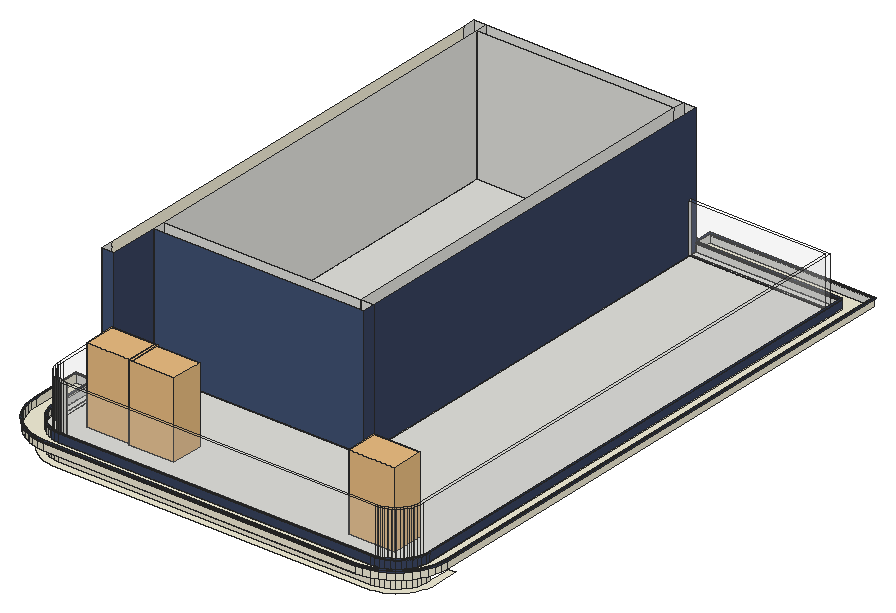
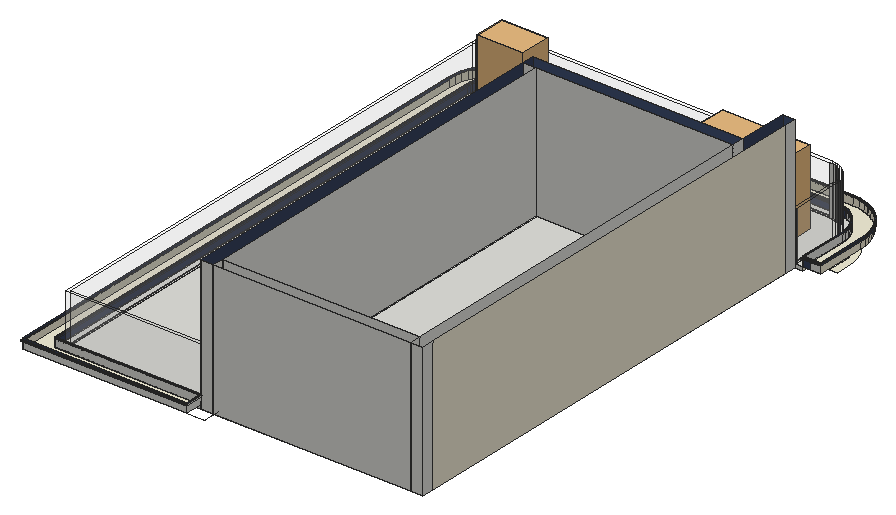
# SketchUp Ruby script. Lengths in inches.
U = 1.inch
M = Sketchup.active_model
def pt(a) = Geom::Point3d.new(a.map { |v| v * U })
def face(e, loops, mat)
  f = e.add_face(loops[0].map { |a| pt(a) })
  loops[1..].each { |l| e.add_face(l.map { |a| pt(a) }).erase! }
  f.material = f.back_material = mat if mat
  f
end
# faces: each face lists its corners as indices into pts; further lists are holes
def faces(e, pts, list, mat = nil) = list.each { |f| face(e, (f[0].is_a?(Array) ? f : [f]).map { |l| l.map { |i| pts[i] } }, mat) }
# xy, xz, yz: faces in a plane at the given z, y or x. An outline is a flat list of corners, or four numbers for a rectangle; further outlines are holes
def ring(l) = l.size == 4 ? [[l[0], l[1]], [l[2], l[1]], [l[2], l[3]], [l[0], l[3]]] : l.each_slice(2).to_a
def flat(e, list, mat, &to3) = list.each { |f| face(e, (f[0].is_a?(Array) ? f : [f]).map { |l| ring(l).map { |u, v| to3.(u, v) } }, mat) }
def xy(e, z, list, mat = nil) = flat(e, list, mat) { |x, y| [x, y, z] }
def xz(e, y, list, mat = nil) = flat(e, list, mat) { |x, z| [x, y, z] }
def yz(e, x, list, mat = nil) = flat(e, list, mat) { |y, z| [x, y, z] }
def lines(e, pts, list) = list.each { |a, b| e.add_line(pt(pts[a]), pt(pts[b])) }
# prism: a flat outline (further loops are holes) pulled along v
def prism(e, loops, v, mat = nil)
  f = face(e, loops, mat); d = Geom::Vector3d.new(v.map { |x| x * U })
  f.pushpull(f.normal.samedirection?(d) ? d.length : -d.length)
end
def box(e, o, s, mat = nil) = prism(e, [[o, [o[0] + s[0], o[1], o[2]], [o[0] + s[0], o[1] + s[1], o[2]], [o[0], o[1] + s[1], o[2]]]], [0, 0, s[2]], mat)
def at(x, y, z, deg = 0) = Geom::Transformation.translation(pt([x, y, z])) * Geom::Transformation.rotation(ORIGIN, Z_AXIS, deg.degrees)
def axes(o, x, y, z) = Geom::Transformation.new([*x, 0, *y, 0, *z, 0, *pt(o).to_a, 1])
def part(name) = M.definitions.add(name)
# library, detail: a bought-in or finely detailed component or shape, given as its bounding box
def library(name, o, s) = part(name).tap { |d| box(d.entities, o, s) }
def detail(e, o, s) = box(e.add_group.entities, o, s)
def put(e, d, t, mat = nil) = e.add_instance(d, t).tap { |i| i.material = mat if mat }
def group(e, t, mat = nil) = e.add_group.tap { |g| g.transformation = t; g.material = mat if mat }.entities
root = M.entities
M.materials.add("0359 AP 9643 Sailor’s Stripes-N").color = [65, 82, 115]
M.materials.add("0360 AP 9644 Monsoon Midnight-N").color = [56, 67, 95]
M.materials.add("0905 AP 7844 MILD YELLOW").color = [242, 237, 215]
M.materials.add("Glass Clear 001").color = [246, 246, 246]
M.materials["Glass Clear 001"].alpha = 0.1
c1 = library("Ficus triangularis Variegata 002",[-17,-11.8,0.01],[33.04,22.7,54.61])
xy(root,253.9375,[[134.66,24.81,360,24.81,363.8,25.06,367.54,25.8,371.15,27.03,374.56,28.71,377.73,30.83,380.6,33.34,383.11,36.2,385.23,39.37,386.91,42.79,388.14,46.4,388.88,50.14,389.13,53.9375,389.13,71.07,384,71.07,384,53.9375,383.79,50.8,383.18,47.73,382.17,44.75,380.78,41.9375,379.04,39.33,376.97,36.97,374.61,34.9,372,33.15,369.18,31.76,366.21,30.76,363.13,30.14,360,29.9375,134.95,29.9375,131.9375,30.29,128.99,31.02,126.8125,31.86,126.15,32.11,123.48,33.56,121.01,35.33,118.78,37.4,116.84,39.73,115.2,42.29,113.9,45.03,112.95,47.92,112.38,50.91,112.1875,53.9375,112.1875,65.19,107.06,65.19,107.06,53.78,107.28,50.26,107.98,46.63,109.125,43.13,110.7,39.8,112.69,36.69,115.06,33.86,117.76,31.35,120.76,29.2,124,27.45,124.96,27.08,127.44,26.12,131.02,25.23]],"0905 AP 7844 MILD YELLOW")
xy(root,264,[[134.95,29.9375,131.9375,30.29,128.99,31.02,126.8125,31.86,126.15,32.11,123.48,33.56,121.01,35.33,118.78,37.4,116.84,39.73,115.2,42.29,113.9,45.03,112.95,47.92,112.38,50.91,112.1875,53.9375,112.1875,89.9375,126.8125,89.9375,126.8125,125.9375,278.3125,125.9375,278.3125,425.9375,384,425.9375,384,53.9375,383.79,50.8,383.18,47.73,382.17,44.75,380.78,41.9375,379.04,39.33,376.97,36.97,374.61,34.9,372,33.15,369.18,31.76,366.21,30.76,363.13,30.14,360,29.9375],[117.8125,89.9375,126.8125,425.9375],[126.8125,125.9375,278.3125,134.9375],[126.8125,134.9375,269.3125,417.55],[269.3125,134.9375,278.3125,425.9375],
  [126.8125,417.55,269.3125,425.9375]])
xy(root,266.6875,[[134.95,29.9375,360,29.9375,363.13,30.14,366.21,30.76,369.18,31.76,372,33.15,374.61,34.9,376.97,36.97,379.04,39.33,380.78,41.9375,382.17,44.75,383.18,47.73,383.79,50.8,384,53.9375,384,425.9375,278.3125,425.9375,278.3125,421.33,379.39,421.33,379.39,53.9375,379.23,51.41,378.73,48.92,377.92,46.52,376.79,44.24,375.39,42.13,373.71,40.23,371.81,38.55,369.7,37.14,367.42,36.02,365.02,35.21,362.53,34.71,360,34.55,135.22,34.55,132.76,34.83,130.375,35.42,128.47,36.16,128.09,36.31,125.93,37.47,123.93,38.9,122.13,40.57,120.5625,42.46,119.24,44.53,118.1875,46.74,117.42,49.08,116.96,51.49,116.8,54.08,116.8,89.9375,112.1875,89.9375,112.1875,53.9375,112.38,50.91,112.95,47.92,113.9,45.03,115.2,42.29,116.84,39.73,118.78,37.4,121.01,35.33,123.48,33.56,126.15,32.11,126.8125,31.86,128.99,31.02,131.9375,30.29],[135.22,34.55,132.76,34.83,130.375,35.42,128.47,36.16,128.09,36.31,125.93,37.47,123.93,38.9,122.13,40.57,120.5625,42.46,119.24,44.53,118.1875,46.74,117.42,49.08,116.96,51.49,116.8,54.08,116.8,89.9375,118.94,89.9375,118.94,54.15,119.09,51.76,119.5,49.62,120.18,47.54,121.12,45.57,122.29,43.73,123.69,42.05,125.29,40.57,127.07,39.3,128.99,38.26,129.25,38.16,131.02,37.47,133.14,36.95,135.35,36.69,360,36.69,362.25,36.84,364.46,37.28,366.6,38,368.625,39,370.5,40.25,372.2,41.74,373.68,43.4375,374.9375,45.3125,375.93,47.34,376.66,49.47,377.1,51.6875,377.25,53.9375,377.25,419.18,278.3125,419.18,278.3125,421.33,379.39,421.33,379.39,53.9375,379.23,51.41,378.73,48.92,377.92,46.52,376.79,44.24,375.39,42.13,373.71,40.23,371.81,38.55,369.7,37.14,367.42,36.02,365.02,35.21,362.53,34.71,360,34.55],[135.35,36.69,360,36.69,362.25,36.84,364.46,37.28,366.6,38,368.625,39,370.5,40.25,372.2,41.74,373.68,43.4375,374.9375,45.3125,375.93,47.34,376.66,49.47,377.1,51.6875,377.25,53.9375,377.25,419.18,278.3125,419.18,278.3125,125.9375,126.8125,125.9375,126.8125,89.9375,118.94,89.9375,118.94,54.15,119.09,51.76,119.5,49.62,120.18,47.54,121.12,45.57,122.29,43.73,123.69,42.05,125.29,40.57,127.07,39.3,128.99,38.26,129.25,38.16,131.02,37.47,133.14,36.95]])
xy(root,266.6875,[[134.21,17.08,129.64,17.61,125.11,18.73,122.17,19.87,120.76,20.42,116.65,22.63,112.86,25.35,109.4375,28.53,106.45,32.11,103.93,36.04,101.93,40.26,100.48,44.7,99.6,49.28,99.33,53.53,99.33,89.9375,112.1875,89.9375,112.1875,53.9375,112.38,50.91,112.95,47.92,113.9,45.03,115.2,42.29,116.84,39.73,118.78,37.4,121.01,35.33,123.48,33.56,126.15,32.11,126.8125,31.86,128.99,31.02,131.9375,30.29,134.95,29.9375,360,29.9375,363.13,30.14,366.21,30.76,369.18,31.76,372,33.15,374.61,34.9,376.97,36.97,379.04,39.33,380.78,41.9375,382.17,44.75,383.18,47.73,383.79,50.8,384,53.9375,384,425.9375,278.3125,425.9375,278.3125,438.8,396.86,438.8,396.86,53.9375,396.54,49.125,395.6,44.4,394.05,39.83,391.92,35.51,389.24,31.5,386.0625,27.875,382.4375,24.7,378.43,22.02,374.11,19.88,369.54,18.34,364.8125,17.39,360,17.08]],"0905 AP 7844 MILD YELLOW")
xy(root,272.125,[[[134.16,16.27,129.49,16.81,124.86,17.96,121.88,19.11,120.41,19.68,116.22,21.94,112.34,24.72,108.85,27.97,105.79,31.63,103.22,35.65,101.17,39.96,99.69,44.49,98.79,49.18,98.52,53.5,98.52,90.75,113,90.75,113,53.96,113.1875,51.01,113.74,48.125,114.65,45.34,115.91,42.68,117.49,40.21,119.375,37.96,121.53,35.96,123.91,34.25,126.49,32.85,127.11,32.62,129.23,31.8,132.08,31.09,135,30.75,360,30.75,363.03,30.95,366,31.54,368.875,32.52,371.59,33.86,374.12,35.54,376.4,37.54,378.4,39.82,380.08,42.34,381.42,45.0625,382.4,47.9375,382.99,50.91,383.1875,53.9375,383.1875,425.125,277.5,425.125,277.5,439.61,397.67,439.61,397.67,53.9375,397.35,49.02,396.39,44.1875,394.8,39.52,392.625,35.1,389.89,31,386.64,27.3,382.93,24.05,378.84,21.3125,374.42,19.13,369.75,17.55,364.92,16.59,360,16.27],[134.21,17.08,360,17.08,364.8125,17.39,369.54,18.34,374.11,19.88,378.43,22.02,382.4375,24.7,386.0625,27.875,389.24,31.5,391.92,35.51,394.05,39.83,395.6,44.4,396.54,49.125,396.86,53.9375,396.86,438.8,278.3125,438.8,278.3125,425.9375,384,425.9375,384,53.9375,383.79,50.8,383.18,47.73,382.17,44.75,380.78,41.9375,379.04,39.33,376.97,36.97,374.61,34.9,372,33.15,369.18,31.76,366.21,30.76,363.13,30.14,360,29.9375,134.95,29.9375,131.9375,30.29,128.99,31.02,126.8125,31.86,126.15,32.11,123.48,33.56,121.01,35.33,118.78,37.4,116.84,39.73,115.2,42.29,113.9,45.03,112.95,47.92,112.38,50.91,112.1875,53.9375,112.1875,89.9375,99.33,89.9375,99.33,53.53,99.6,49.28,100.48,44.7,101.93,40.26,103.93,36.04,106.45,32.11,109.4375,28.53,112.86,25.35,116.65,22.63,120.76,20.42,122.17,19.87,125.11,18.73,129.64,17.61]]],"0360 AP 9644 Monsoon Midnight-N")
xy(root,272.8125,[[[134.16,16.27,360,16.27,364.92,16.59,369.75,17.55,374.42,19.13,378.84,21.3125,382.93,24.05,386.64,27.3,389.89,31,392.625,35.1,394.8,39.52,396.39,44.1875,397.35,49.02,397.67,53.9375,397.67,439.61,277.5,439.61,277.5,425.125,383.1875,425.125,383.1875,53.9375,382.99,50.91,382.4,47.9375,381.42,45.0625,380.08,42.34,378.4,39.82,376.4,37.54,374.12,35.54,371.59,33.86,368.875,32.52,366,31.54,363.03,30.95,360,30.75,135,30.75,132.08,31.09,129.23,31.8,127.11,32.62,126.49,32.85,123.91,34.25,121.53,35.96,119.375,37.96,117.49,40.21,115.91,42.68,114.65,45.34,113.74,48.125,113.1875,51.01,113,53.96,113,90.75,98.52,90.75,98.52,53.5,98.79,49.18,99.69,44.49,101.17,39.96,103.22,35.65,105.79,31.63,108.85,27.97,112.34,24.72,116.22,21.94,120.41,19.68,121.88,19.11,124.86,17.96,129.49,16.81],[134.21,17.08,129.64,17.61,125.11,18.73,122.17,19.87,120.76,20.42,116.65,22.63,112.86,25.35,109.4375,28.53,106.45,32.11,103.93,36.04,101.93,40.26,100.48,44.7,99.6,49.28,99.33,53.53,99.33,89.9375,112.1875,89.9375,112.1875,53.9375,112.38,50.91,112.95,47.92,113.9,45.03,115.2,42.29,116.84,39.73,118.78,37.4,121.01,35.33,123.48,33.56,126.15,32.11,126.8125,31.86,128.99,31.02,131.9375,30.29,134.95,29.9375,360,29.9375,363.13,30.14,366.21,30.76,369.18,31.76,372,33.15,374.61,34.9,376.97,36.97,379.04,39.33,380.78,41.9375,382.17,44.75,383.18,47.73,383.79,50.8,384,53.9375,384,425.9375,278.3125,425.9375,278.3125,438.8,396.86,438.8,396.86,53.9375,396.54,49.125,395.6,44.4,394.05,39.83,391.92,35.51,389.24,31.5,386.0625,27.875,382.4375,24.7,378.43,22.02,374.11,19.88,369.54,18.34,364.8125,17.39,360,17.08]]],"0360 AP 9644 Monsoon Midnight-N")
xz(root,16.27,[[134.16,272.125,360,272.8125]],"0360 AP 9644 Monsoon Midnight-N")
xz(root,17.08,[[134.21,272.125,360,272.8125],[134.21,272.8125,360,273.625]],"0360 AP 9644 Monsoon Midnight-N")
xz(root,17.08,[[134.21,266.6875,360,272.125]],"0905 AP 7844 MILD YELLOW")
xz(root,29.9375,[[134.95,266.6875,360,272.125],[134.95,272.125,360,272.8125],[134.95,272.8125,360,273.625]],"0360 AP 9644 Monsoon Midnight-N")
xz(root,29.9375,[[134.95,253.9375,360,264],[134.95,264,360,266.6875]],"0905 AP 7844 MILD YELLOW")
xz(root,30.75,[[135,272.125,360,272.8125]],"0360 AP 9644 Monsoon Midnight-N")
xz(root,34.55,[[135.22,266.6875,360,302.6875]],"Glass Clear 001")
xz(root,36.69,[[135.35,266.6875,360,302.6875]],"Glass Clear 001")
xz(root,89.9375,[[112.1875,264,117.8125,266.6875],[117.8125,264,126.8125,266.6875],[99.33,266.6875,106.59,272.125],[116.8,266.6875,117.8125,302.6875],[117.8125,266.6875,118.94,302.6875],
  [106.59,272.125,112.1875,272.8125]])
xz(root,89.9375,[[118.94,266.6875,126.8125,266.6875,126.8125,360,117.8125,360,117.8125,303.4375,118.94,303.4375]],"0359 AP 9643 Sailor’s Stripes-N")
xz(root,89.9375,[[106.59,266.6875,112.1875,272.125],[99.33,272.125,106.59,272.8125],[99.33,272.8125,106.59,273.625],[106.59,272.8125,112.1875,273.625]],"0360 AP 9644 Monsoon Midnight-N")
xz(root,90.75,[[98.52,272.125,106.59,272.8125],[106.59,272.125,113,272.8125]])
xz(root,125.9375,[[126.8125,264,278.3125,266.6875]])
xz(root,125.9375,[[126.8125,266.6875,278.3125,360]],"0359 AP 9643 Sailor’s Stripes-N")
xz(root,134.9375,[[126.8125,264,269.3125,360],[269.3125,264,278.3125,360]])
xz(root,417.55,[[126.8125,264,269.3125,360]])
xz(root,419.18,[[278.3125,266.6875,377.25,302.6875]],"Glass Clear 001")
xz(root,421.33,[[278.3125,266.6875,379.39,302.6875]],"Glass Clear 001")
xz(root,425.125,[[277.5,272.125,383.1875,272.8125]])
xz(root,425.9375,[[117.8125,264,126.8125,360],[126.8125,264,269.3125,360],[269.3125,264,278.3125,360],[278.3125,264,384,266.6875],[278.3125,266.6875,384,272.125]])
xz(root,425.9375,[[278.3125,272.125,384,272.8125],[278.3125,272.8125,384,273.625]],"0360 AP 9644 Monsoon Midnight-N")
xz(root,438.8,[[278.3125,266.6875,396.86,272.125]])
xz(root,438.8,[[278.3125,272.125,396.86,272.8125],[278.3125,272.8125,396.86,273.625]],"0360 AP 9644 Monsoon Midnight-N")
xz(root,439.61,[[277.5,272.125,397.67,272.8125]])
yz(root,98.52,[[53.5,272.125,90.75,272.8125]],"0360 AP 9644 Monsoon Midnight-N")
yz(root,99.33,[[53.53,272.125,89.9375,272.8125],[53.53,272.8125,89.9375,273.625]],"0360 AP 9644 Monsoon Midnight-N")
yz(root,99.33,[[53.53,266.6875,89.9375,272.125]],"0905 AP 7844 MILD YELLOW")
yz(root,112.1875,[[53.9375,266.6875,89.9375,272.125]])
yz(root,112.1875,[[53.9375,272.125,89.9375,272.8125],[53.9375,272.8125,89.9375,273.625]],"0360 AP 9644 Monsoon Midnight-N")
yz(root,112.1875,[[53.9375,264,89.9375,266.6875]],"0905 AP 7844 MILD YELLOW")
yz(root,113,[[53.96,272.125,90.75,272.8125]])
yz(root,116.8,[[54.08,266.6875,89.9375,302.6875]],"Glass Clear 001")
yz(root,117.8125,[[89.9375,264,98.79,360],[416.9375,264,425.9375,360]])
yz(root,117.8125,[[98.79,264,416.9375,360]],"0905 AP 7844 MILD YELLOW")
yz(root,118.94,[[54.15,266.6875,89.9375,302.6875]],"Glass Clear 001")
yz(root,126.8125,[[89.9375,264,125.9375,266.6875],[125.9375,264,134.9375,360],[134.9375,264,417.55,360],[417.55,264,425.9375,360]])
yz(root,126.8125,[[89.9375,266.6875,125.9375,360]],"0360 AP 9644 Monsoon Midnight-N")
yz(root,269.3125,[[134.9375,264,417.55,360],[417.55,264,425.9375,360]])
yz(root,277.5,[[425.125,272.125,439.61,272.8125]])
yz(root,278.3125,[[125.9375,264,134.9375,266.6875],[134.9375,264,425.9375,266.6875],[419.18,266.6875,421.33,302.6875],[425.9375,266.6875,438.8,272.125]])
yz(root,278.3125,[[125.9375,266.6875,134.9375,360],[134.9375,266.6875,419.18,266.6875,419.18,303.4375,421.33,303.4375,421.33,266.6875,425.9375,266.6875,425.9375,360,134.9375,360],[425.9375,272.125,438.8,272.8125],[425.9375,272.8125,438.8,273.625]],"0360 AP 9644 Monsoon Midnight-N")
yz(root,377.25,[[53.9375,266.6875,419.18,302.6875]],"Glass Clear 001")
yz(root,379.39,[[53.9375,266.6875,421.33,302.6875]],"Glass Clear 001")
yz(root,383.1875,[[53.9375,272.125,425.125,272.8125]],"0360 AP 9644 Monsoon Midnight-N")
yz(root,384,[[53.9375,266.6875,425.9375,272.125],[53.9375,272.125,425.9375,272.8125],[53.9375,272.8125,425.9375,273.625]],"0360 AP 9644 Monsoon Midnight-N")
yz(root,384,[[53.9375,264,425.9375,266.6875]],"0905 AP 7844 MILD YELLOW")
yz(root,396.86,[[53.9375,272.125,438.8,272.8125],[53.9375,272.8125,438.8,273.625]],"0360 AP 9644 Monsoon Midnight-N")
yz(root,396.86,[[53.9375,266.6875,438.8,272.125]],"0905 AP 7844 MILD YELLOW")
yz(root,397.67,[[53.9375,272.125,439.61,272.8125]],"0360 AP 9644 Monsoon Midnight-N")
p = [[134.95,29.9375,264],[131.9375,30.29,264],[131.9375,30.29,253.9375],[134.95,29.9375,253.9375],[363.13,30.14,264],[360,29.9375,264],
  [360,29.9375,253.9375],[363.13,30.14,253.9375],[366.21,30.76,264],[366.21,30.76,253.9375],[128.99,31.02,264],[128.99,31.02,253.9375],
  [369.18,31.76,264],[369.18,31.76,253.9375],[126.8125,31.86,264],[126.8125,31.86,253.9375],[372,33.15,264],[372,33.15,253.9375],
  [126.15,32.11,264],[126.15,32.11,253.9375],[123.48,33.56,264],[123.48,33.56,253.9375],[374.61,34.9,264],[374.61,34.9,253.9375],
  [121.01,35.33,264],[121.01,35.33,253.9375],[376.97,36.97,264],[376.97,36.97,253.9375],[118.78,37.4,264],[118.78,37.4,253.9375],
  [379.04,39.33,264],[379.04,39.33,253.9375],[116.84,39.73,264],[116.84,39.73,253.9375],[380.78,41.9375,264],[380.78,41.9375,253.9375],
  [115.2,42.29,264],[115.2,42.29,253.9375],[382.17,44.75,264],[382.17,44.75,253.9375],[113.9,45.03,264],[113.9,45.03,253.9375],
  [383.18,47.73,264],[383.18,47.73,253.9375],[112.95,47.92,264],[112.95,47.92,253.9375],[383.79,50.8,264],[383.79,50.8,253.9375],
  [112.38,50.91,264],[112.38,50.91,253.9375],[384,53.9375,264],[384,53.9375,253.9375],[112.1875,53.9375,264],[112.1875,53.9375,253.9375],
  [134.95,29.9375,266.6875],[131.9375,30.29,266.6875],[363.13,30.14,266.6875],[360,29.9375,266.6875],[366.21,30.76,266.6875],[128.99,31.02,266.6875],
  [369.18,31.76,266.6875],[126.8125,31.86,266.6875],[372,33.15,266.6875],[126.15,32.11,266.6875],[123.48,33.56,266.6875],[374.61,34.9,266.6875],
  [121.01,35.33,266.6875],[376.97,36.97,266.6875],[118.78,37.4,266.6875],[379.04,39.33,266.6875],[116.84,39.73,266.6875],[380.78,41.9375,266.6875],
  [115.2,42.29,266.6875],[382.17,44.75,266.6875],[113.9,45.03,266.6875],[383.18,47.73,266.6875],[112.95,47.92,266.6875],[383.79,50.8,266.6875],
  [112.38,50.91,266.6875],[384,53.9375,266.6875],[112.1875,53.9375,266.6875],[129.64,17.61,266.6875],[134.21,17.08,266.6875],[134.21,17.08,272.125],
  [129.64,17.61,272.125],[360,17.08,266.6875],[364.8125,17.39,266.6875],[364.8125,17.39,272.125],[360,17.08,272.125],[369.54,18.34,266.6875],
  [369.54,18.34,272.125],[125.11,18.73,266.6875],[125.11,18.73,272.125],[374.11,19.88,266.6875],[374.11,19.88,272.125],[122.17,19.87,266.6875],
  [122.17,19.87,272.125],[120.76,20.42,266.6875],[120.76,20.42,272.125],[378.43,22.02,266.6875],[378.43,22.02,272.125],[116.65,22.63,266.6875],
  [116.65,22.63,272.125],[382.4375,24.7,266.6875],[382.4375,24.7,272.125],[112.86,25.35,266.6875],[112.86,25.35,272.125],[386.0625,27.875,266.6875],
  [386.0625,27.875,272.125],[109.4375,28.53,266.6875],[109.4375,28.53,272.125],[389.24,31.5,266.6875],[389.24,31.5,272.125],[106.45,32.11,266.6875],
  [106.45,32.11,272.125],[131.9375,30.29,272.125],[134.95,29.9375,272.125],[360,29.9375,272.125],[363.13,30.14,272.125],[366.21,30.76,272.125],
  [128.99,31.02,272.125],[369.18,31.76,272.125],[126.8125,31.86,272.125],[391.92,35.51,266.6875],[391.92,35.51,272.125],[372,33.15,272.125],
  [126.15,32.11,272.125],[103.93,36.04,266.6875],[103.93,36.04,272.125],[123.48,33.56,272.125],[374.61,34.9,272.125],[121.01,35.33,272.125],
  [132.76,34.83,266.6875],[135.22,34.55,266.6875],[135.22,34.55,302.6875],[132.76,34.83,302.6875],[360,34.55,266.6875],[362.53,34.71,266.6875],
  [362.53,34.71,302.6875],[360,34.55,302.6875],[365.02,35.21,266.6875],[365.02,35.21,302.6875],[130.375,35.42,266.6875],[130.375,35.42,302.6875],
  [376.97,36.97,272.125],[367.42,36.02,266.6875],[367.42,36.02,302.6875],[118.78,37.4,272.125],[128.47,36.16,266.6875],[128.47,36.16,302.6875],
  [394.05,39.83,266.6875],[394.05,39.83,272.125],[101.93,40.26,266.6875],[101.93,40.26,272.125],[369.7,37.14,266.6875],[369.7,37.14,302.6875],
  [128.09,36.31,266.6875],[128.09,36.31,302.6875],[125.93,37.47,266.6875],[125.93,37.47,302.6875],[135.35,36.69,266.6875],[133.14,36.95,266.6875],
  [133.14,36.95,302.6875],[135.35,36.69,302.6875],[362.25,36.84,266.6875],[360,36.69,266.6875],[360,36.69,302.6875],[362.25,36.84,302.6875],
  [364.46,37.28,266.6875],[364.46,37.28,302.6875],[131.02,37.47,266.6875],[131.02,37.47,302.6875],[379.04,39.33,272.125],[371.81,38.55,266.6875],
  [371.81,38.55,302.6875],[366.6,38,266.6875],[366.6,38,302.6875],[116.84,39.73,272.125],[123.93,38.9,266.6875],[123.93,38.9,302.6875],
  [129.25,38.16,266.6875],[129.25,38.16,302.6875],[368.625,39,266.6875],[368.625,39,302.6875],[128.99,38.26,266.6875],[128.99,38.26,302.6875],
  [127.07,39.3,266.6875],[127.07,39.3,302.6875],[373.71,40.23,266.6875],[373.71,40.23,302.6875],[122.13,40.57,266.6875],[122.13,40.57,302.6875],
  [370.5,40.25,266.6875],[370.5,40.25,302.6875],[125.29,40.57,266.6875],[125.29,40.57,302.6875],[380.78,41.9375,272.125],[115.2,42.29,272.125],
  [395.6,44.4,266.6875],[395.6,44.4,272.125],[375.39,42.13,266.6875],[375.39,42.13,302.6875],[100.48,44.7,266.6875],[100.48,44.7,272.125],
  [372.2,41.74,266.6875],[372.2,41.74,302.6875],[120.5625,42.46,266.6875],[120.5625,42.46,302.6875],[123.69,42.05,266.6875],[123.69,42.05,302.6875],
  [373.68,43.4375,266.6875],[373.68,43.4375,302.6875],[382.17,44.75,272.125],[122.29,43.73,266.6875],[122.29,43.73,302.6875],[376.79,44.24,266.6875],
  [376.79,44.24,302.6875],[113.9,45.03,272.125],[119.24,44.53,266.6875],[119.24,44.53,302.6875],[374.9375,45.3125,266.6875],[374.9375,45.3125,302.6875],
  [121.12,45.57,266.6875],[121.12,45.57,302.6875],[377.92,46.52,266.6875],[377.92,46.52,302.6875],[396.54,49.125,266.6875],[396.54,49.125,272.125],
  [118.1875,46.74,266.6875],[118.1875,46.74,302.6875],[99.6,49.28,266.6875],[99.6,49.28,272.125],[383.18,47.73,272.125],[112.95,47.92,272.125],
  [375.93,47.34,266.6875],[375.93,47.34,302.6875],[120.18,47.54,266.6875],[120.18,47.54,302.6875],[378.73,48.92,266.6875],[378.73,48.92,302.6875],
  [117.42,49.08,266.6875],[117.42,49.08,302.6875],[376.66,49.47,266.6875],[376.66,49.47,302.6875],[119.5,49.62,266.6875],[119.5,49.62,302.6875],
  [383.79,50.8,272.125],[112.38,50.91,272.125],[379.23,51.41,266.6875],[379.23,51.41,302.6875],[116.96,51.49,266.6875],[116.96,51.49,302.6875],
  [396.86,53.9375,266.6875],[396.86,53.9375,272.125],[99.33,53.53,266.6875],[99.33,53.53,272.125],[377.1,51.6875,266.6875],[377.1,51.6875,302.6875],
  [119.09,51.76,266.6875],[119.09,51.76,302.6875],[384,53.9375,272.125],[112.1875,53.9375,272.125],[379.39,53.9375,266.6875],[379.39,53.9375,302.6875],
  [116.8,54.08,266.6875],[116.8,54.08,302.6875],[377.25,53.9375,266.6875],[377.25,53.9375,302.6875],[118.94,54.15,266.6875],[118.94,54.15,302.6875],
  [129.49,16.81,272.125],[134.16,16.27,272.125],[134.16,16.27,272.8125],[129.49,16.81,272.8125],[360,16.27,272.125],[364.92,16.59,272.125],
  [364.92,16.59,272.8125],[360,16.27,272.8125],[369.75,17.55,272.125],[369.75,17.55,272.8125],[124.86,17.96,272.125],[124.86,17.96,272.8125],
  [134.21,17.08,272.8125],[129.64,17.61,272.8125],[364.8125,17.39,272.8125],[360,17.08,272.8125],[369.54,18.34,272.8125],[125.11,18.73,272.8125],
  [374.42,19.13,272.125],[374.42,19.13,272.8125],[121.88,19.11,272.125],[121.88,19.11,272.8125],[374.11,19.88,272.8125],[122.17,19.87,272.8125],
  [120.41,19.68,272.125],[120.41,19.68,272.8125],[378.84,21.3125,272.125],[378.84,21.3125,272.8125],[116.22,21.94,272.125],[116.22,21.94,272.8125],
  [120.76,20.42,272.8125],[378.43,22.02,272.8125],[116.65,22.63,272.8125],[382.93,24.05,272.125],[382.93,24.05,272.8125],[112.34,24.72,272.125],
  [112.34,24.72,272.8125],[382.4375,24.7,272.8125],[112.86,25.35,272.8125],[386.64,27.3,272.125],[386.64,27.3,272.8125],[108.85,27.97,272.125],
  [108.85,27.97,272.8125],[386.0625,27.875,272.8125],[109.4375,28.53,272.8125],[389.89,31,272.125],[389.89,31,272.8125],[389.24,31.5,272.8125],
  [105.79,31.63,272.125],[105.79,31.63,272.8125],[106.45,32.11,272.8125],[131.9375,30.29,272.8125],[134.95,29.9375,272.8125],[360,29.9375,272.8125],
  [363.13,30.14,272.8125],[366.21,30.76,272.8125],[128.99,31.02,272.8125],[135,30.75,272.125],[132.08,31.09,272.125],[132.08,31.09,272.8125],
  [135,30.75,272.8125],[363.03,30.95,272.125],[360,30.75,272.125],[360,30.75,272.8125],[363.03,30.95,272.8125],[369.18,31.76,272.8125],
  [366,31.54,272.125],[366,31.54,272.8125],[126.8125,31.86,272.8125],[392.625,35.1,272.125],[392.625,35.1,272.8125],[129.23,31.8,272.125],
  [129.23,31.8,272.8125],[368.875,32.52,272.125],[368.875,32.52,272.8125],[391.92,35.51,272.8125],[103.22,35.65,272.125],[103.22,35.65,272.8125],
  [127.11,32.62,272.125],[127.11,32.62,272.8125],[372,33.15,272.8125],[126.15,32.11,272.8125],[103.93,36.04,272.8125],[123.48,33.56,272.8125],
  [371.59,33.86,272.125],[371.59,33.86,272.8125],[126.49,32.85,272.125],[126.49,32.85,272.8125],[123.91,34.25,272.125],[123.91,34.25,272.8125],
  [374.61,34.9,272.8125],[121.01,35.33,272.8125],[374.12,35.54,272.125],[374.12,35.54,272.8125],[121.53,35.96,272.125],[121.53,35.96,272.8125],
  [376.97,36.97,272.8125],[394.8,39.52,272.125],[394.8,39.52,272.8125],[118.78,37.4,272.8125],[376.4,37.54,272.125],[376.4,37.54,272.8125],
  [394.05,39.83,272.8125],[101.17,39.96,272.125],[101.17,39.96,272.8125],[101.93,40.26,272.8125],[119.375,37.96,272.125],[119.375,37.96,272.8125],
  [379.04,39.33,272.8125],[116.84,39.73,272.8125],[378.4,39.82,272.125],[378.4,39.82,272.8125],[117.49,40.21,272.125],[117.49,40.21,272.8125],
  [380.78,41.9375,272.8125],[396.39,44.1875,272.125],[396.39,44.1875,272.8125],[115.2,42.29,272.8125],[380.08,42.34,272.125],[380.08,42.34,272.8125],
  [395.6,44.4,272.8125],[99.69,44.49,272.125],[99.69,44.49,272.8125],[115.91,42.68,272.125],[115.91,42.68,272.8125],[100.48,44.7,272.8125],
  [382.17,44.75,272.8125],[113.9,45.03,272.8125],[381.42,45.0625,272.125],[381.42,45.0625,272.8125],[114.65,45.34,272.125],[114.65,45.34,272.8125],
  [397.35,49.02,272.125],[397.35,49.02,272.8125],[396.54,49.125,272.8125],[98.79,49.18,272.125],[98.79,49.18,272.8125],[99.6,49.28,272.8125],
  [383.18,47.73,272.8125],[112.95,47.92,272.8125],[382.4,47.9375,272.125],[382.4,47.9375,272.8125],[113.74,48.125,272.125],[113.74,48.125,272.8125],
  [383.79,50.8,272.8125],[112.38,50.91,272.8125],[382.99,50.91,272.125],[382.99,50.91,272.8125],[113.1875,51.01,272.125],[113.1875,51.01,272.8125],
  [397.67,53.9375,272.125],[397.67,53.9375,272.8125],[396.86,53.9375,272.8125],[98.52,53.5,272.125],[98.52,53.5,272.8125],[99.33,53.53,272.8125],
  [384,53.9375,272.8125],[112.1875,53.9375,272.8125],[383.1875,53.9375,272.125],[383.1875,53.9375,272.8125],[113,53.96,272.125],[113,53.96,272.8125],
  [134.21,17.08,273.625],[129.64,17.61,273.625],[364.8125,17.39,273.625],[360,17.08,273.625],[369.54,18.34,273.625],[125.11,18.73,273.625],
  [374.11,19.88,273.625],[122.17,19.87,273.625],[120.76,20.42,273.625],[378.43,22.02,273.625],[116.65,22.63,273.625],[382.4375,24.7,273.625],
  [112.86,25.35,273.625],[386.0625,27.875,273.625],[109.4375,28.53,273.625],[389.24,31.5,273.625],[106.45,32.11,273.625],[131.9375,30.29,273.625],
  [134.95,29.9375,273.625],[360,29.9375,273.625],[363.13,30.14,273.625],[366.21,30.76,273.625],[128.99,31.02,273.625],[369.18,31.76,273.625],
  [126.8125,31.86,273.625],[391.92,35.51,273.625],[372,33.15,273.625],[126.15,32.11,273.625],[103.93,36.04,273.625],[123.48,33.56,273.625],
  [374.61,34.9,273.625],[121.01,35.33,273.625],[376.97,36.97,273.625],[118.78,37.4,273.625],[394.05,39.83,273.625],[101.93,40.26,273.625],
  [379.04,39.33,273.625],[116.84,39.73,273.625],[380.78,41.9375,273.625],[115.2,42.29,273.625],[395.6,44.4,273.625],[100.48,44.7,273.625],
  [382.17,44.75,273.625],[113.9,45.03,273.625],[396.54,49.125,273.625],[99.6,49.28,273.625],[383.18,47.73,273.625],[112.95,47.92,273.625],
  [383.79,50.8,273.625],[112.38,50.91,273.625],[396.86,53.9375,273.625],[99.33,53.53,273.625],[384,53.9375,273.625],[112.1875,53.9375,273.625],
  [265.45,438.8,266.6875],[265.45,138.8,266.6875],[278.3125,438.8,266.6875]]
faces(root,p,[[0,1,2,3],[4,5,6,7],[8,4,7,9],[1,10,11,2],[12,8,9,13],[10,14,15,11],[16,12,13,17],[14,18,19,15],
  [18,20,21,19],[22,16,17,23],[20,24,25,21],[26,22,23,27],[24,28,29,25],[30,26,27,31],[28,32,33,29],[34,30,31,35],
  [32,36,37,33],[38,34,35,39],[36,40,41,37],[42,38,39,43],[40,44,45,41],[46,42,43,47],[44,48,49,45],[50,46,47,51],
  [48,52,53,49],[1,0,54,55],[5,4,56,57],[4,8,58,56],[10,1,55,59],[8,12,60,58],[14,10,59,61],[12,16,62,60],
  [18,14,61,63],[20,18,63,64],[16,22,65,62],[24,20,64,66],[22,26,67,65],[28,24,66,68],[26,30,69,67],[32,28,68,70],
  [30,34,71,69],[36,32,70,72],[34,38,73,71],[40,36,72,74],[38,42,75,73],[44,40,74,76],[42,46,77,75],[48,44,76,78],
  [46,50,79,77],[52,48,78,80],[81,82,83,84],[85,86,87,88],[86,89,90,87],[91,81,84,92],[89,93,94,90],[95,91,92,96],
  [97,95,96,98],[93,99,100,94],[101,97,98,102],[99,103,104,100],[105,101,102,106],[103,107,108,104],[109,105,106,110],[107,111,112,108],
  [113,109,110,114],[111,123,124,112],[127,113,114,128],[123,150,151,124],[152,127,128,153],[150,198,199,151],[202,152,153,203],[198,226,227,199],
  [230,202,203,231],[226,252,253,227],[254,230,231,255]],"0905 AP 7844 MILD YELLOW")
faces(root,p,[[54,55,115,116],[56,57,117,118],[58,56,118,119],[55,59,120,115],[60,58,119,121],[59,61,122,120],[62,60,121,125],[65,62,125,130],
  [67,65,130,144],[69,67,144,172],[71,69,172,196],[73,71,196,212],[75,73,212,232],[77,75,232,246],[79,77,246,260],[270,271,272,273],
  [274,275,276,277],[275,278,279,276],[280,270,273,281],[282,283,84,83],[284,285,88,87],[286,284,87,90],[283,287,92,84],[278,288,289,279],
  [290,280,281,291],[292,286,90,94],[287,293,96,92],[294,290,291,295],[288,296,297,289],[298,294,295,299],[293,300,98,96],[301,292,94,100],
  [300,302,102,98],[296,303,304,297],[305,298,299,306],[307,301,100,104],[302,308,106,102],[303,309,310,304],[311,305,306,312],[313,307,104,108],
  [308,314,110,106],[309,315,316,310],[317,313,108,112],[318,311,312,319],[314,320,114,110],[321,322,116,115],[323,324,118,117],[324,325,119,118],
  [326,321,115,120],[327,328,329,330],[331,332,333,334],[325,335,121,119],[336,331,334,337],[338,326,120,122],[315,339,340,316],[328,341,342,329],
  [343,336,337,344],[345,317,112,124],[346,318,319,347],[341,348,349,342],[335,350,125,121],[351,338,122,126],[320,352,128,114],[353,351,126,129],
  [354,343,344,355],[348,356,357,349],[356,358,359,357],[350,360,130,125],[361,353,129,131],[362,354,355,363],[358,364,365,359],[360,366,144,130],
  [339,367,368,340],[369,361,131,147],[370,362,363,371],[372,345,124,151],[373,346,347,374],[352,375,153,128],[364,376,377,365],[366,378,172,144],
  [379,369,147,177],[380,370,371,381],[376,382,383,377],[378,384,196,172],[367,385,386,368],[387,379,177,197],[388,380,381,389],[390,372,151,199],
  [391,373,374,392],[382,393,394,383],[375,395,203,153],[384,396,212,196],[397,387,197,217],[398,388,389,399],[393,400,401,394],[385,402,403,386],
  [404,390,199,227],[405,391,392,406],[395,407,231,203],[396,408,232,212],[409,397,217,233],[410,398,399,411],[400,412,413,401],[408,414,246,232],
  [415,409,233,247],[416,410,411,417],[412,418,419,413],[402,420,421,403],[422,404,227,253],[423,405,406,424],[407,425,255,231],[414,426,260,246],
  [427,415,247,261],[428,416,417,429],[418,430,431,419],[283,282,432,433],[285,284,434,435],[284,286,436,434],[287,283,433,437],[286,292,438,436],
  [293,287,437,439],[300,293,439,440],[292,301,441,438],[302,300,440,442],[301,307,443,441],[308,302,442,444],[307,313,445,443],[314,308,444,446],
  [313,317,447,445],[320,314,446,448],[322,321,449,450],[324,323,451,452],[325,324,452,453],[321,326,454,449],[335,325,453,455],[326,338,456,454],
  [317,345,457,447],[350,335,455,458],[338,351,459,456],[352,320,448,460],[351,353,461,459],[360,350,458,462],[353,361,463,461],[366,360,462,464],
  [361,369,465,463],[345,372,466,457],[375,352,460,467],[378,366,464,468],[369,379,469,465],[384,378,468,470],[379,387,471,469],[372,390,472,466],
  [395,375,467,473],[396,384,470,474],[387,397,475,471],[390,404,476,472],[407,395,473,477],[408,396,474,478],[397,409,479,475],[414,408,478,480],
  [409,415,481,479],[404,422,482,476],[425,407,477,483],[426,414,480,484],[415,427,485,481]],"0360 AP 9644 Monsoon Midnight-N")
faces(root,p,[[61,63,126,122],[63,64,129,126],[64,66,131,129],[66,68,147,131],[160,161,162,163],[161,170,171,162],[68,70,177,147],[170,180,181,171],
  [70,72,197,177],[72,74,217,197],[74,76,233,217],[76,78,247,233],[78,80,261,247]])
faces(root,p,[[132,133,134,135],[136,137,138,139],[137,140,141,138],[142,132,135,143],[140,145,146,141],[148,142,143,149],[145,154,155,146],[156,148,149,157],
  [158,156,157,159],[164,165,166,167],[168,164,167,169],[154,173,174,155],[175,168,169,176],[178,158,159,179],[182,175,176,183],[180,184,185,181],
  [184,186,187,185],[173,188,189,174],[190,178,179,191],[192,182,183,193],[186,194,195,187],[188,200,201,189],[204,192,193,205],[206,190,191,207],
  [194,208,209,195],[210,204,205,211],[208,213,214,209],[200,215,216,201],[218,206,207,219],[220,210,211,221],[213,222,223,214],[215,224,225,216],
  [228,218,219,229],[234,220,221,235],[222,236,237,223],[224,238,239,225],[240,228,229,241],[242,234,235,243],[236,244,245,237],[238,248,249,239],
  [250,240,241,251],[256,242,243,257],[244,258,259,245],[248,262,263,249],[264,250,251,265],[266,256,257,267],[258,268,269,259]],"Glass Clear 001")
lines(root,p,[[486,487],[488,486]])
put(root,c1,at(153.14,65.49,266.6875))
put(root,c1,at(183.96,64.59,266.6875))
put(root,c1,at(345.48,61.79,266.6875))
